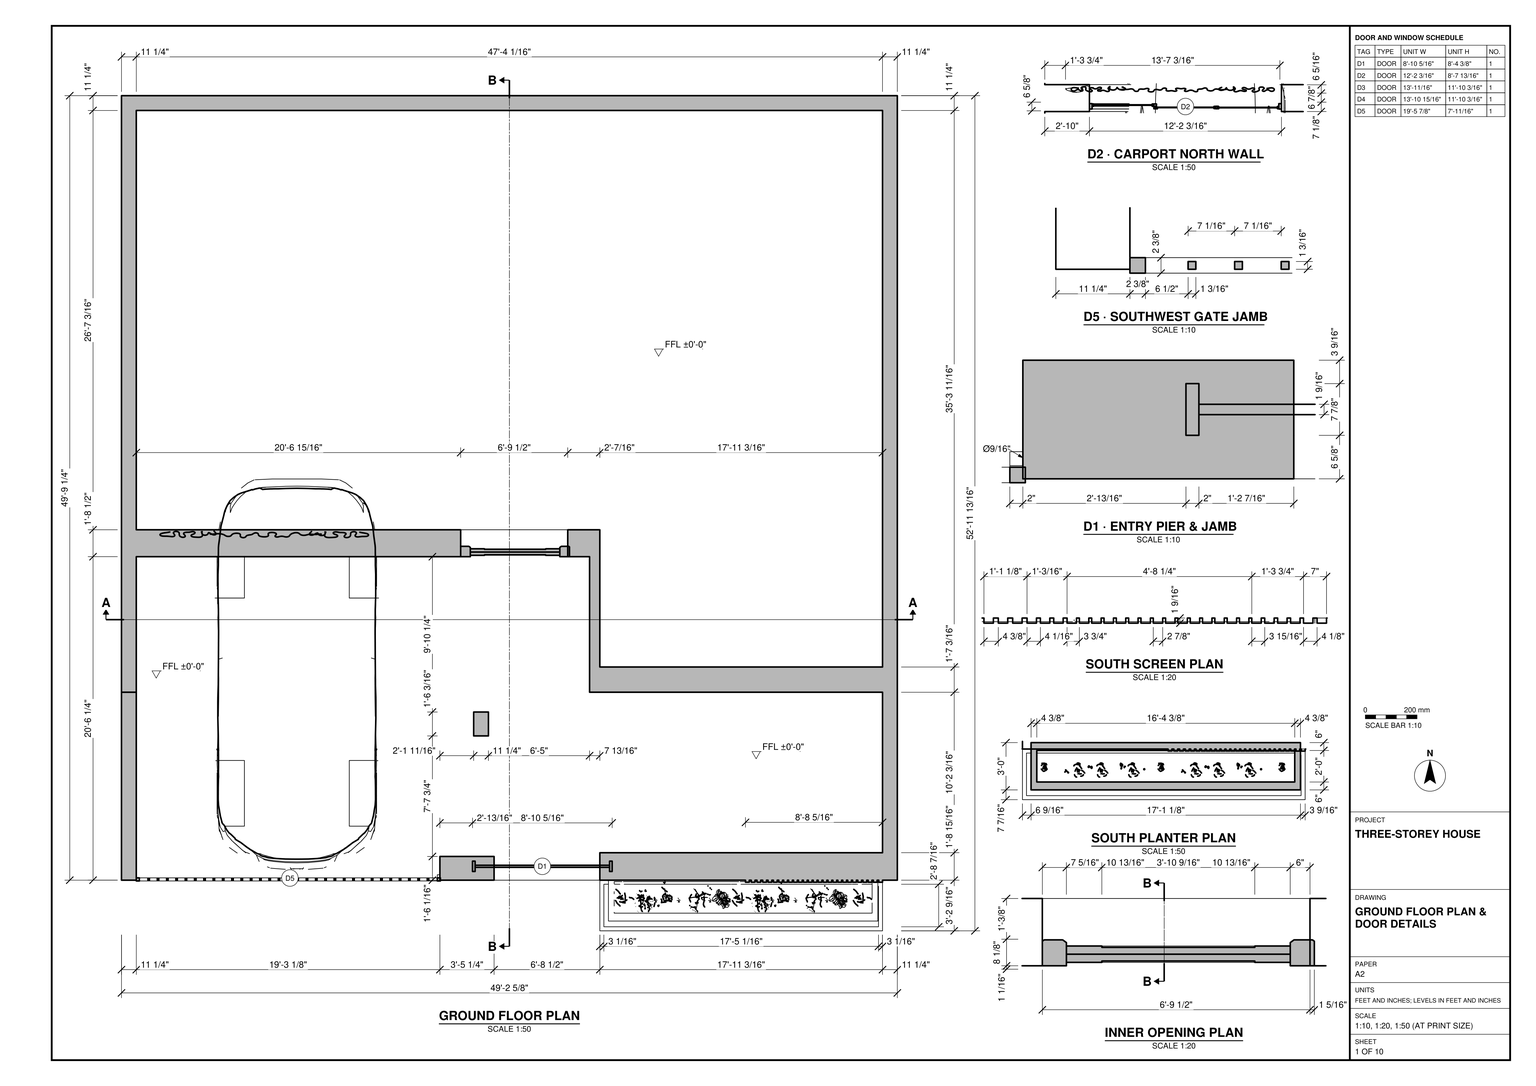
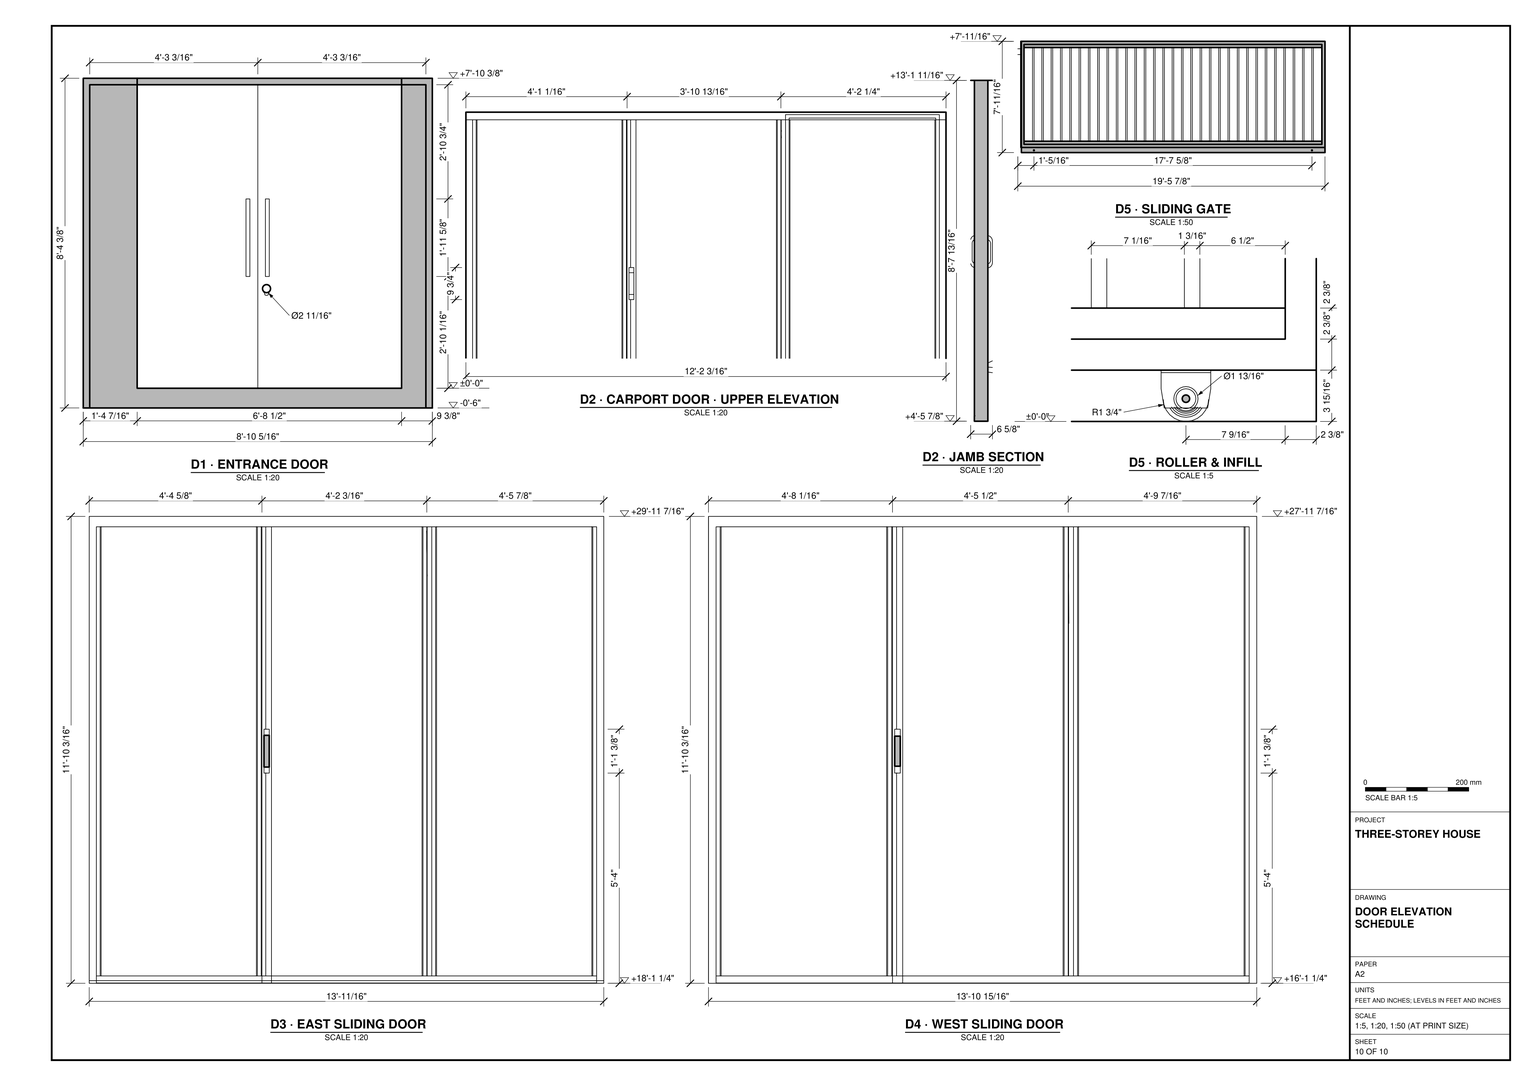
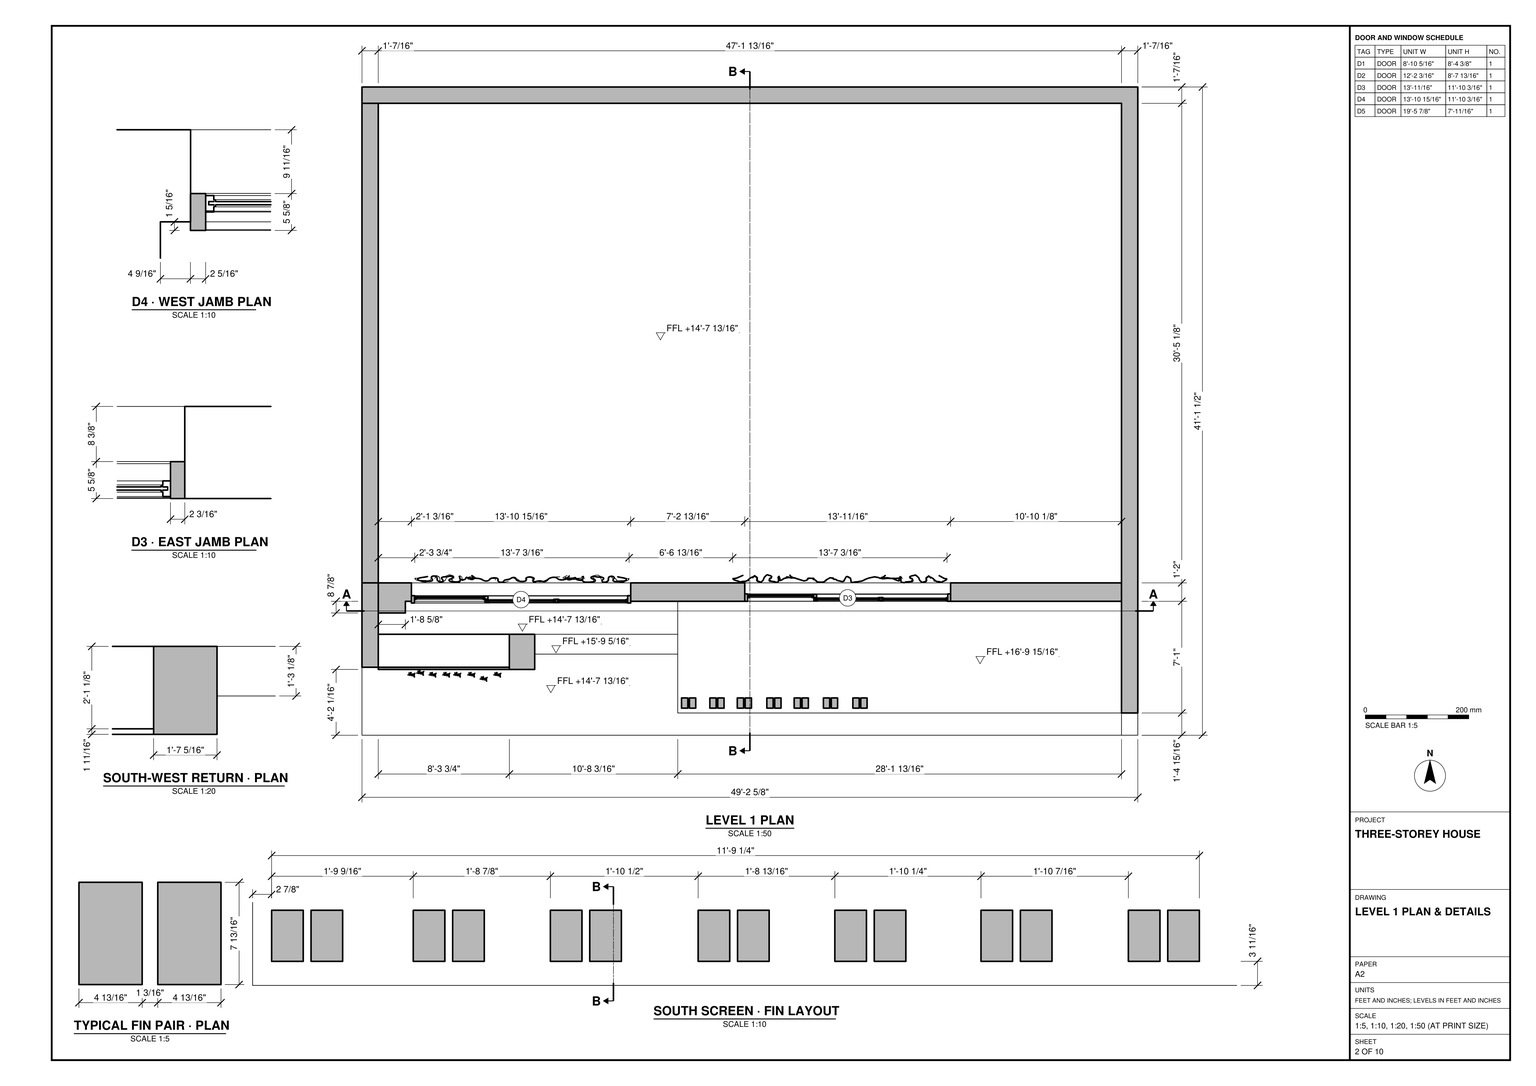
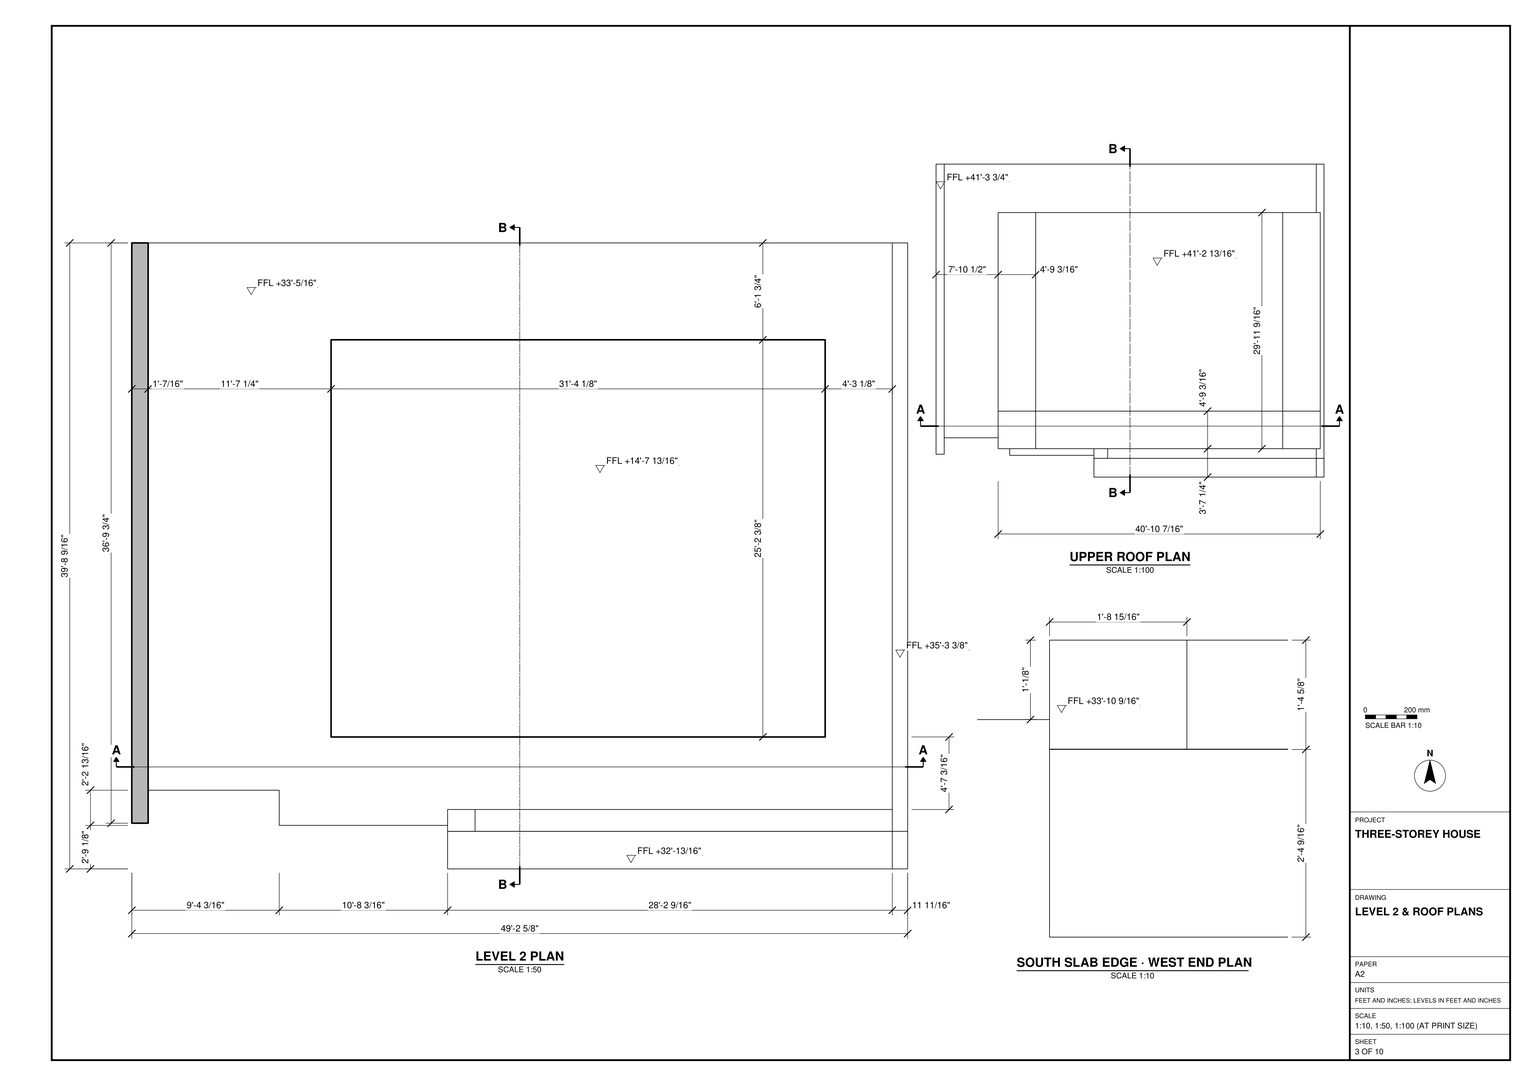
Build the three-storey house in SketchUp from task_files/diagram_01.pdf. Work in feet and inches. Set out the full model to measure 49'-2 5/8" across the frontage, 52'-11 13/16" from front to back and 41'-9 3/4" high. Use the finished floor levels ±0'-0", +14'-7 13/16" and +33'-5/16".

Use the south frontage to align the plans. Place the carport at the southwest, with its sliding gate facing the street, the separate entrance to its east and the projecting planter farther east. Follow the drawn wall thicknesses, returns and opening positions rather than using a uniform wall thickness throughout. Fit the entrance leaves, carport door, sliding doors and gate to their respective openings using the plan details and door elevations.

On the level above the carport, set the wall with the east and west sliding doors back from the terrace edge. Model the changes in terrace level, the southwest return and the paired vertical screen fins. Follow the plans and sections for the floor slabs, roof profile, and any stairs, built-in joinery or main furniture shown. Place a car in the carport and planting in the south planter. Decor and loose items may be any suitable library components.

Keep shell elements and individual furniture or joinery pieces in separate groups or components, and use components for repeated parts. Save one SketchUp model as output_files/three_storey_house_with_a_carport_and_screened_terrace.skp.

# SketchUp Ruby script. Lengths in inches.
U = 1.inch
M = Sketchup.active_model
def pt(a) = Geom::Point3d.new(a.map { |v| v * U })
def face(e, loops, mat)
  f = e.add_face(loops[0].map { |a| pt(a) })
  loops[1..].each { |l| e.add_face(l.map { |a| pt(a) }).erase! }
  f.material = f.back_material = mat if mat
  f
end
# faces: each face lists its corners as indices into pts; further lists are holes
def faces(e, pts, list, mat = nil) = list.each { |f| face(e, (f[0].is_a?(Array) ? f : [f]).map { |l| l.map { |i| pts[i] } }, mat) }
# xy, xz, yz: faces in a plane at the given z, y or x. An outline is a flat list of corners, or four numbers for a rectangle; further outlines are holes
def ring(l) = l.size == 4 ? [[l[0], l[1]], [l[2], l[1]], [l[2], l[3]], [l[0], l[3]]] : l.each_slice(2).to_a
def flat(e, list, mat, &to3) = list.each { |f| face(e, (f[0].is_a?(Array) ? f : [f]).map { |l| ring(l).map { |u, v| to3.(u, v) } }, mat) }
def xy(e, z, list, mat = nil) = flat(e, list, mat) { |x, y| [x, y, z] }
def xz(e, y, list, mat = nil) = flat(e, list, mat) { |x, z| [x, y, z] }
def yz(e, x, list, mat = nil) = flat(e, list, mat) { |y, z| [x, y, z] }
def lines(e, pts, list) = list.each { |a, b| e.add_line(pt(pts[a]), pt(pts[b])) }
# prism: a flat outline (further loops are holes) pulled along v
def prism(e, loops, v, mat = nil)
  f = face(e, loops, mat); d = Geom::Vector3d.new(v.map { |x| x * U })
  f.pushpull(f.normal.samedirection?(d) ? d.length : -d.length)
end
def box(e, o, s, mat = nil) = prism(e, [[o, [o[0] + s[0], o[1], o[2]], [o[0] + s[0], o[1] + s[1], o[2]], [o[0], o[1] + s[1], o[2]]]], [0, 0, s[2]], mat)
def at(x, y, z, deg = 0) = Geom::Transformation.translation(pt([x, y, z])) * Geom::Transformation.rotation(ORIGIN, Z_AXIS, deg.degrees)
def axes(o, x, y, z) = Geom::Transformation.new([*x, 0, *y, 0, *z, 0, *pt(o).to_a, 1])
def part(name) = M.definitions.add(name)
# library, detail: a bought-in or finely detailed component or shape, given as its bounding box
def library(name, o, s) = part(name).tap { |d| box(d.entities, o, s) }
def detail(e, o, s) = box(e.add_group.entities, o, s)
def put(e, d, t, mat = nil) = e.add_instance(d, t).tap { |i| i.material = mat if mat }
def group(e, t, mat = nil) = e.add_group.tap { |g| g.transformation = t; g.material = mat if mat }.entities
root = M.entities
M.materials.add("Material__1").color = [95, 70, 46]
M.materials.add("[0130_Gainsboro]").color = [220, 220, 220]
M.materials.add("[0132_LightGray]").color = [169, 169, 169]
M.materials.add("[Field Rectangle Tile]").color = [196, 189, 179]
M.materials.add("[Granite Dark Gray]").color = [69, 68, 68]
M.materials.add("[Wood Veneer 01]").color = [120, 70, 37]
c1 = library("Group5_1",[-7.56,-66.38,0.11],[6.33,135.04,120.95])
c2 = library("Sliding Door",[0,0,0],[94.49,5.83,91.73])
c3 = library("元件\#5",[-4.39,0,0],[5.37,35.83,90.55])
c4 = library("2016+Honda+Civic+LX+Sedan+(1)",[0.01,0.03,0.02],[16.17,34.46,10.62])
c5 = library("Sliding Gate",[0,0,0],[194.88,4.13,70.58])
c6 = library("door (3)",[-4.72,-1.97,0],[7.87,106.3,100.39])
c7 = library("Potted trailing plant",[-13.52,-13.75,-7.41],[40.56,40.5625,37.31])
c8 = library("Areca palm plant",[0,0,0],[49.1,36.6,54.46])
c9 = library("Group\#74",[-84.69,-90.07,-0.36],[176.51,175.13,171.4])
c10 = library("Group38\#2",[14.01,28.44,-23.43],[18.58,18.32,38.89])
c11 = library("Group20\#1",[-20.81,-17.08,3.79],[39.86,39.43,37.51])
c12 = library("Group\#130",[-7.34,-1.2,0],[38.67,35.81,49.04])
xy(root,-6,[[0,38.5625,590.625,635.8125]])
xy(root,0,[[364.15,0,579.35,38.5625],[[11.28,38.5625,242.39,38.5625,242.39,56.625,283.64,56.625,283.64,38.5625,364.15,38.5625,364.15,59.47,579.35,59.47,579.35,181.65,356.34,181.65,356.34,284.84,339.71,284.84,339.71,305.33,258.21,305.33,258.21,284.84,11.28,284.84],[268.1,148.39,279.35,166.59]],[0,181.65,11.28,181.65,11.28,284.84,258.21,284.84,258.21,305.33,11.28,305.33,11.28,624.53,579.35,624.53,579.35,200.85,364.15,200.85,364.15,305.33,339.71,305.33,339.71,284.84,356.34,284.84,356.34,181.65,590.625,181.65,590.625,635.8125,0,635.8125],[364.15,200.85,579.35,200.85,579.35,624.53,11.28,624.53,11.28,305.33,364.15,305.33],[364.15,200.85,579.35,200.85,579.35,624.53,11.28,624.53,11.28,305.33,364.15,305.33]])
xy(root,7.6875,[[367.23,3.08,576.27,3.08,576.27,33.92,574.36,33.92,574.36,35.49,367.23,35.49]])
xy(root,33.625,[[[364.15,0,579.35,0,579.35,37,576.47,37,576.47,38.5625,575.22,38.5625,575.22,37,572.35,37,572.35,38.5625,571.28,38.5625,571.28,37,568.41,37,568.41,38.5625,567.35,38.5625,567.35,37,564.47,37,564.47,38.5625,563.41,38.5625,563.41,37,560.53,37,560.53,38.5625,559.47,38.5625,559.47,37,556.6,37,556.6,38.5625,555.72,38.5625,555.72,37,552.85,37,552.85,38.5625,551.97,38.5625,551.97,37,549.1,37,549.1,38.5625,548.22,38.5625,548.22,37,545.35,37,545.35,38.5625,544.47,38.5625,544.47,37,541.6,37,541.6,38.5625,540.72,38.5625,540.72,37,537.85,37,537.85,38.5625,536.97,38.5625,536.97,37,534.1,37,534.1,38.5625,533.22,38.5625,533.22,37,530.35,37,530.35,38.5625,529.47,38.5625,529.47,37,526.6,37,526.6,38.5625,525.72,38.5625,525.72,37,522.85,37,522.85,38.5625,521.97,38.5625,521.97,37,519.1,37,519.1,38.5625,518.22,38.5625,518.22,37,515.35,37,515.35,38.5625,514.47,38.5625,514.47,37,511.6,37,511.6,38.5625,510.72,38.5625,510.72,37,507.85,37,507.85,38.5625,506.97,38.5625,506.97,37,504.1,37,504.1,38.5625,503.22,38.5625,503.22,37,500.35,37,500.35,38.5625,499.16,38.5625,499.16,37,496.28,37,496.28,38.5625,495.1,38.5625,495.1,37,492.22,37,492.22,38.5625,491.03,38.5625,491.03,37,488.16,37,488.16,38.5625,486.66,38.5625,486.66,37,483.78,37,483.78,38.5625,482.28,38.5625,482.28,37,479.41,37,479.41,38.5625,477.91,38.5625,477.91,37,475.03,37,475.03,38.5625,364.15,38.5625],[367.23,3.08,367.23,35.49,574.36,35.49,574.36,33.92,576.27,33.92,576.27,3.08]],[475.03,37,477.91,38.5625],[479.41,37,482.28,38.5625],[483.78,37,486.66,38.5625],[488.16,37,491.03,38.5625],
  [492.22,37,495.1,38.5625],[496.28,37,499.16,38.5625],[500.35,37,503.22,38.5625],[504.1,37,506.97,38.5625],[507.85,37,510.72,38.5625],
  [511.6,37,514.47,38.5625],[515.35,37,518.22,38.5625],[519.1,37,521.97,38.5625],[522.85,37,525.72,38.5625],[526.6,37,529.47,38.5625],
  [530.35,37,533.22,38.5625],[534.1,37,536.97,38.5625],[537.85,37,540.72,38.5625],[541.6,37,544.47,38.5625],[545.35,37,548.22,38.5625],
  [549.1,37,551.97,38.5625],[552.85,37,555.72,38.5625],[556.6,37,559.47,38.5625],[560.53,37,563.41,38.5625],[564.47,37,567.35,38.5625],
  [568.41,37,571.28,38.5625],[572.35,37,575.22,38.5625],[576.47,37,579.35,38.5625]])
xy(root,53.59,[[45.25,284.84,191.44,305.33]])
xy(root,106.375,[[475.03,37,477.91,37,477.91,38.5625,479.41,38.5625,479.41,37,482.28,37,482.28,38.5625,483.78,38.5625,483.78,37,486.66,37,486.66,38.5625,488.16,38.5625,488.16,37,491.03,37,491.03,38.5625,492.22,38.5625,492.22,37,495.1,37,495.1,38.5625,496.28,38.5625,496.28,37,499.16,37,499.16,38.5625,500.35,38.5625,500.35,37,503.22,37,503.22,38.5625,504.1,38.5625,504.1,37,506.97,37,506.97,38.5625,507.85,38.5625,507.85,37,510.72,37,510.72,38.5625,511.6,38.5625,511.6,37,514.47,37,514.47,38.5625,515.35,38.5625,515.35,37,518.22,37,518.22,38.5625,519.1,38.5625,519.1,37,521.97,37,521.97,38.5625,522.85,38.5625,522.85,37,525.72,37,525.72,38.5625,526.6,38.5625,526.6,37,529.47,37,529.47,38.5625,530.35,38.5625,530.35,37,533.22,37,533.22,38.5625,534.1,38.5625,534.1,37,536.97,37,536.97,38.5625,537.85,38.5625,537.85,37,540.72,37,540.72,38.5625,541.6,38.5625,541.6,37,544.47,37,544.47,38.5625,545.35,38.5625,545.35,37,548.22,37,548.22,38.5625,549.1,38.5625,549.1,37,551.97,37,551.97,38.5625,552.85,38.5625,552.85,37,555.72,37,555.72,38.5625,556.6,38.5625,556.6,37,559.47,37,559.47,38.5625,560.53,38.5625,560.53,37,563.41,37,563.41,38.5625,564.47,38.5625,564.47,37,567.35,37,567.35,38.5625,568.41,38.5625,568.41,37,571.28,37,571.28,38.5625,572.35,38.5625,572.35,37,575.22,37,575.22,38.5625,576.47,38.5625,576.47,37,579.35,37,579.35,59.47,364.15,59.47,364.15,38.5625,475.03,38.5625],[0,38.5625,11.28,181.65],[242.39,38.5625,283.64,56.625],[579.35,38.5625,590.625,181.65]])
xy(root,155.5625,[[0,148.39,11.28,181.65],[11.28,148.39,11.28,284.84,356.34,284.84,356.34,148.39,279.35,148.39,279.35,166.59,268.1,166.59,268.1,148.39],[356.34,148.39,364.15,181.65],[364.15,148.39,590.625,181.65]])
xy(root,157.25,[[258.21,284.84,339.71,305.33]])
xy(root,157.66,[[45.25,284.84,191.44,305.33]])
xy(root,169.8125,[[[0,181.65,0,635.8125,590.625,635.8125,590.625,181.65,356.34,181.65,356.34,284.84,11.28,284.84,11.28,181.65],[364.15,200.85,579.35,200.85,579.35,624.53,11.28,624.53,11.28,305.33,364.15,305.33]]])
xy(root,171.6875,[[0,142.32,590.625,148.39]])
xy(root,175.8125,[[0,142.32,578.2,142.32,578.2,204.07,131.51,204.07,131.51,192.39,12.42,192.39,12.42,194.07,0,194.07],[578.2,142.32,590.625,219.17],[0,194.07,12.42,258.3],[12.42,219.17,578.2,219.17,578.2,244.27,33.05,244.27,33.05,235.4,12.42,235.4],[578.2,219.17,590.625,244.27],
  [12.42,235.4,33.05,235.4,33.05,244.27,578.2,244.27,578.2,258.3,12.42,258.3],[0,258.3,12.42,303.21],[12.42,258.3,578.2,623.39],[0,303.21,12.42,623.39]])
xy(root,189.28,[[240.375,181.65,285.45,204.07],[285.45,181.65,578.2,204.07],[12.42,194.07,112.2,219.17],[131.51,204.07,240.375,219.17],[240.375,204.07,285.45,219.17],
  [285.45,204.07,578.2,219.17],[240.375,219.17,285.45,244.27],[285.45,219.17,578.2,244.27]])
xy(root,189.28,[[240.375,159.26,285.45,181.65],[285.45,159.26,578.2,181.65]],"[Granite Dark Gray]")
xy(root,189.49,[[578.2,159.26,590.625,181.65],[578.2,181.65,590.625,244.27]])
xy(root,193.23,[[37.65,244.27,204.59,258.3]])
xy(root,201.91,[[[240.375,159.26,578.2,244.27],[243.27,162.92,248.08,170.71],[249.27,162.92,254.08,170.71],[264.83,162.92,269.64,170.71],[270.83,162.92,275.64,170.71],[285.71,162.92,290.52,170.71],[291.71,162.92,296.52,170.71],[308.21,162.92,313.02,170.71],[314.21,162.92,319.02,170.71],[329.02,162.92,333.83,170.71],[335.02,162.92,339.83,170.71],[351.27,162.92,356.08,170.71],[357.27,162.92,362.08,170.71],[373.71,162.92,378.52,170.71],[379.71,162.92,384.52,170.71]]])
xy(root,218.08,[[291.41,244.27,448.1,258.3]])
xy(root,233.16,[[12.42,194.07,112.2,219.17]])
xy(root,235.85,[[12.42,192.39,112.2,194.07]])
xy(root,335.41,[[37.65,244.27,204.59,258.3]])
xy(root,359.46,[[291.41,244.27,448.1,258.3]])
xy(root,369.9375,[[[240.375,159.26,578.2,187.89],[485.96,166.9,487.51,167.125,488.95,167.74,490.18,168.71,491.12,169.97,491.7,171.42,491.88,172.98,491.66,174.53,491.04,175.97,490.07,177.2,488.82,178.13,487.36,178.71,485.81,178.9,484.26,178.67,482.82,178.06,481.59,177.09,480.65,175.83,480.07,174.38,479.88,172.82,480.11,171.27,480.73,169.83,481.69,168.6,482.95,167.67,484.4,167.08],[393.96,166.9,395.51,167.125,396.95,167.74,398.18,168.71,399.12,169.97,399.7,171.42,399.88,172.98,399.66,174.53,399.04,175.97,398.07,177.2,396.82,178.13,395.36,178.71,393.81,178.9,392.26,178.67,390.82,178.06,389.59,177.09,388.65,175.83,388.07,174.38,387.88,172.82,388.11,171.27,388.73,169.83,389.69,168.6,390.95,167.67,392.4,167.08],[243.27,162.92,248.08,170.71],[249.27,162.92,254.08,170.71],[264.83,162.92,269.64,170.71],[270.83,162.92,275.64,170.71],[285.71,162.92,290.52,170.71],[291.71,162.92,296.52,170.71],[308.21,162.92,313.02,170.71],[314.21,162.92,319.02,170.71],[329.02,162.92,333.83,170.71],[335.02,162.92,339.83,170.71],[351.27,162.92,356.08,170.71],[357.27,162.92,362.08,170.71],[373.71,162.92,378.52,170.71],[379.71,162.92,384.52,170.71]]])
xy(root,372.63,[[240.375,159.26,578.2,161.57],[578.2,159.26,579.125,161.57]])
xy(root,372.8125,[[393.96,166.9,392.4,167.08,390.95,167.67,389.69,168.6,388.73,169.83,388.11,171.27,387.88,172.82,388.07,174.38,388.65,175.83,389.59,177.09,390.82,178.06,392.26,178.67,393.81,178.9,395.36,178.71,396.82,178.13,398.07,177.2,399.04,175.97,399.66,174.53,399.88,172.98,399.7,171.42,399.12,169.97,398.18,168.71,396.95,167.74,395.51,167.125],[485.96,166.9,484.4,167.08,482.95,167.67,481.69,168.6,480.73,169.83,480.11,171.27,479.88,172.82,480.07,174.38,480.65,175.83,481.59,177.09,482.82,178.06,484.26,178.67,485.81,178.9,487.36,178.71,488.82,178.13,490.07,177.2,491.04,175.97,491.66,174.53,491.88,172.98,491.7,171.42,491.12,169.97,490.18,168.71,488.95,167.74,487.51,167.125]])
xy(root,378.8125,[[578.2,181.65,590.625,187.89],[578.2,187.89,578.2,623.39,0,623.39,0,635.8125,590.625,635.8125,590.625,187.89],[240.375,187.89,240.375,192.39,131.51,192.39,131.51,219.17,12.42,219.17,12.42,235.4,22.74,235.4,22.74,227.71,238.08,227.71,238.08,235.4,33.05,235.4,33.05,244.27,578.2,244.27,578.2,187.89],[0,219.17,12.42,258.3],[22.74,227.71,25.42,235.4],
  [25.42,227.71,238.08,235.4],[12.42,235.4,12.42,258.3,578.2,258.3,578.2,244.27,33.05,244.27,33.05,235.4],[0,258.3,12.42,303.21],[12.42,258.3,578.2,623.39],[0,303.21,12.42,623.39]])
xy(root,381.44,[[240.375,159.26,578.91,161.57],[578.91,159.26,579.125,161.57]])
xy(root,384.8125,[[240.375,159.26,578.91,187.84],[240.375,187.84,578.91,187.89],[261.29,187.89,578.91,204.48],[0,219.17,12.42,635.8125]])
xy(root,396.3125,[[240.375,187.89,261.29,204.48],[[112.2,192.39,240.375,192.39,240.375,204.48,578.91,204.48,578.91,635.8125,12.42,635.8125,12.42,219.17,112.2,219.17],[151.68,259.69,527.8,562.07]]])
xy(root,406.5625,[[240.375,187.84,261.29,204.48]])
xy(root,423.375,[[578.91,159.26,590.625,187.89],[578.91,187.89,590.625,635.8125]])
xy(root,475.25,[[117.45,225.46,117.45,539.13,128.74,539.13,128.74,236.76,550.74,236.76,550.74,539.13,562.03,539.13,562.03,225.46],[151.68,259.69,527.8,562.07]])
xy(root,475.25,[[[94.52,202.53,94.52,562.07,151.68,562.07,151.68,259.69,527.8,259.69,527.8,562.07,584.97,562.07,584.97,202.53],[117.45,225.46,562.03,225.46,562.03,539.13,550.74,539.13,550.74,236.76,128.74,236.76,128.74,539.13,117.45,539.13]]],"[Wood Veneer 01]")
xy(root,477.58,[[94.52,202.53,101.33,562.07]])
xy(root,479.24,[[101.33,202.53,584.97,209.34]],"[Granite Dark Gray]")
xy(root,479.9,[[583.91,209.34,584.97,562.07]])
xy(root,491.3,[[94.52,209.34,101.33,562.07],[583.91,209.34,584.97,562.07]])
xy(root,491.3,[[94.52,202.53,584.97,209.34]],"[Granite Dark Gray]")
xy(root,494.8125,[[94.52,202.53,151.68,259.69],[527.8,202.53,584.97,259.69],[94.52,259.69,151.68,562.07],[151.68,259.69,527.8,562.07],[527.8,259.69,584.97,562.07]])
xy(root,494.8125,[[151.68,202.53,527.8,259.69]],"[Granite Dark Gray]")
xy(root,495.75,[[0,194.07,12.42,635.8125]])
xz(root,0,[[364.15,0,579.35,33.625]])
xz(root,3.08,[[367.23,7.6875,576.27,33.625]])
xz(root,33.92,[[574.36,7.6875,576.27,33.625]])
xz(root,35.49,[[367.23,7.6875,574.36,33.625]])
xz(root,37,[[475.03,33.625,477.91,106.375],[479.41,33.625,482.28,106.375],[483.78,33.625,486.66,106.375],[488.16,33.625,491.03,106.375],[492.22,33.625,495.1,106.375],
  [496.28,33.625,499.16,106.375],[500.35,33.625,503.22,106.375],[504.1,33.625,506.97,106.375],[507.85,33.625,510.72,106.375],[511.6,33.625,514.47,106.375],
  [515.35,33.625,518.22,106.375],[519.1,33.625,521.97,106.375],[522.85,33.625,525.72,106.375],[526.6,33.625,529.47,106.375],[530.35,33.625,533.22,106.375],
  [534.1,33.625,536.97,106.375],[537.85,33.625,540.72,106.375],[541.6,33.625,544.47,106.375],[545.35,33.625,548.22,106.375],[549.1,33.625,551.97,106.375],
  [552.85,33.625,555.72,106.375],[556.6,33.625,559.47,106.375],[560.53,33.625,563.41,106.375],[564.47,33.625,567.35,106.375],[568.41,33.625,571.28,106.375],
  [572.35,33.625,575.22,106.375],[576.47,33.625,579.35,106.375]],"[Wood Veneer 01]")
xz(root,38.5625,[[0,-6,590.625,-6,590.625,0,283.64,0,283.64,74.62,242.77,74.62,242.77,79.01,283.64,79.01,283.64,106.375,242.39,106.375,242.39,0,11.28,0,11.28,106.375,0,106.375],[364.15,0,579.35,33.625],[579.35,0,590.625,106.375],[364.15,33.625,475.03,106.375]])
xz(root,38.5625,[[242.77,74.62,283.64,79.01]],"[Granite Dark Gray]")
xz(root,38.5625,[[477.91,33.625,479.41,106.375],[482.28,33.625,483.78,106.375],[486.66,33.625,488.16,106.375],[491.03,33.625,492.22,106.375],[495.1,33.625,496.28,106.375],
  [499.16,33.625,500.35,106.375],[503.22,33.625,504.1,106.375],[506.97,33.625,507.85,106.375],[510.72,33.625,511.6,106.375],[514.47,33.625,515.35,106.375],
  [518.22,33.625,519.1,106.375],[521.97,33.625,522.85,106.375],[525.72,33.625,526.6,106.375],[529.47,33.625,530.35,106.375],[533.22,33.625,534.1,106.375],
  [536.97,33.625,537.85,106.375],[540.72,33.625,541.6,106.375],[544.47,33.625,545.35,106.375],[548.22,33.625,549.1,106.375],[551.97,33.625,552.85,106.375],
  [555.72,33.625,556.6,106.375],[559.47,33.625,560.53,106.375],[563.41,33.625,564.47,106.375],[567.35,33.625,568.41,106.375],[571.28,33.625,572.35,106.375],
  [575.22,33.625,576.47,106.375]],"[Wood Veneer 01]")
xz(root,56.625,[[242.39,0,283.64,106.375]])
xz(root,59.47,[[364.15,0,579.35,106.375]])
xz(root,142.32,[[0,171.6875,590.625,175.8125]],"[Granite Dark Gray]")
xz(root,148.39,[[268.1,0,279.35,0,279.35,155.5625,590.625,155.5625,590.625,171.6875,0,171.6875,0,155.5625,268.1,155.5625]],"[Granite Dark Gray]")
xz(root,159.26,[[578.2,189.49,590.625,189.49,590.625,423.375,578.91,423.375,578.91,381.44,579.125,381.44,579.125,372.63,578.2,372.63]])
xz(root,159.26,[[240.375,189.28,578.2,201.91],[240.375,369.9375,578.2,372.63],[240.375,381.44,578.91,384.8125]],"[Granite Dark Gray]")
xz(root,161.57,[[240.375,372.63,579.125,381.44]],"[Granite Dark Gray]")
xz(root,162.92,[[243.27,201.91,248.08,369.9375],[249.27,201.91,254.08,369.9375],[264.83,201.91,269.64,369.9375],[270.83,201.91,275.64,369.9375],[285.71,201.91,290.52,369.9375],
  [291.71,201.91,296.52,369.9375],[308.21,201.91,313.02,369.9375],[314.21,201.91,319.02,369.9375],[329.02,201.91,333.83,369.9375],[335.02,201.91,339.83,369.9375],
  [351.27,201.91,356.08,369.9375],[357.27,201.91,362.08,369.9375],[373.71,201.91,378.52,369.9375],[379.71,201.91,384.52,369.9375]],"[Wood Veneer 01]")
xz(root,166.59,[[268.1,0,279.35,155.5625]])
xz(root,170.71,[[243.27,201.91,248.08,369.9375],[249.27,201.91,254.08,369.9375],[264.83,201.91,269.64,369.9375],[270.83,201.91,275.64,369.9375],[285.71,201.91,290.52,369.9375],
  [291.71,201.91,296.52,369.9375],[308.21,201.91,313.02,369.9375],[314.21,201.91,319.02,369.9375],[329.02,201.91,333.83,369.9375],[335.02,201.91,339.83,369.9375],
  [351.27,201.91,356.08,369.9375],[357.27,201.91,362.08,369.9375],[373.71,201.91,378.52,369.9375],[379.71,201.91,384.52,369.9375]])
xz(root,181.65,[[0,0,11.28,106.375],[356.34,0,364.15,155.5625],[0,106.375,11.28,155.5625],[0,155.5625,11.28,169.8125],[356.34,155.5625,364.15,169.8125],
  [364.15,155.5625,590.625,169.8125]])
xz(root,181.65,[[364.15,0,579.35,0,579.35,106.375,590.625,106.375,590.625,155.5625,364.15,155.5625]],"[Field Rectangle Tile]")
xz(root,187.84,[[240.375,384.8125,578.91,384.8125,578.91,416.875,261.29,406.5625,240.375,406.5625]],"[0132_LightGray]")
xz(root,187.89,[[240.375,369.9375,578.2,378.8125],[240.375,384.8125,261.29,396.3125]])
xz(root,192.39,[[112.2,175.8125,131.51,175.8125,131.51,378.8125,240.375,378.8125,240.375,396.3125,112.2,396.3125]],"[0132_LightGray]")
xz(root,192.39,[[12.42,175.8125,112.2,235.85]],"[Granite Dark Gray]")
xz(root,194.07,[[12.42,175.8125,112.2,189.28],[12.42,189.28,112.2,233.16],[12.42,233.16,112.2,235.85]])
xz(root,194.07,[[0,175.8125,12.42,495.75]],"[0132_LightGray]")
xz(root,200.85,[[364.15,0,579.35,169.8125]])
xz(root,202.53,[[94.52,475.25,584.97,475.25,584.97,479.24,101.33,479.24,101.33,477.58,94.52,477.58],[94.52,491.3,584.97,494.8125]],"[Granite Dark Gray]")
xz(root,204.07,[[131.51,175.8125,578.2,189.28]],"[0130_Gainsboro]")
xz(root,204.48,[[261.29,384.8125,578.91,396.3125],[240.375,396.3125,240.375,406.5625,261.29,406.5625,578.91,416.875,578.91,396.3125]])
xz(root,209.34,[[101.33,479.24,584.97,479.24,584.97,479.9,583.91,479.9,583.91,491.3,101.33,491.3]],"[Granite Dark Gray]")
xz(root,219.17,[[12.42,175.8125,12.42,189.28,112.2,189.28,112.2,378.8125,131.51,378.8125,131.51,189.28,578.2,189.28,578.2,175.8125],[12.42,189.28,112.2,233.16],[0,378.8125,12.42,384.8125]])
xz(root,219.17,[[12.42,378.8125,112.2,396.3125]],"[0132_LightGray]")
xz(root,235.4,[[12.42,175.8125,33.05,378.8125]],"[Granite Dark Gray]")
xz(root,244.27,[[578.2,175.8125,590.625,189.49],[240.375,189.28,285.45,201.91]])
xz(root,244.27,[[[33.05,175.8125,578.2,175.8125,578.2,189.28,240.375,189.28,240.375,201.91,578.2,201.91,578.2,378.8125,33.05,378.8125],[37.65,193.23,204.59,335.41],[291.41,218.08,448.1,359.46]]],"[Field Rectangle Tile]")
xz(root,258.3,[[0,175.8125,12.42,378.8125],[[12.42,175.8125,578.2,378.8125],[37.65,193.23,204.59,335.41],[291.41,218.08,448.1,359.46]]])
xz(root,259.69,[[151.68,475.25,527.8,494.8125]])
xz(root,259.69,[[151.68,396.3125,527.8,475.25]],"[0132_LightGray]")
xz(root,284.84,[[339.71,0,356.34,155.5625],[11.28,155.5625,45.25,155.5625,45.25,157.66,191.44,157.66,191.44,155.5625,258.21,155.5625,258.21,157.25,339.71,157.25,339.71,155.5625,356.34,155.5625,356.34,169.8125,11.28,169.8125],[45.25,155.5625,191.44,157.66],[258.21,155.5625,339.71,157.25]])
xz(root,284.84,[[11.28,0,258.21,0,258.21,155.5625,191.44,155.5625,191.44,53.59,45.25,53.59,45.25,155.5625,11.28,155.5625]],"[0130_Gainsboro]")
xz(root,305.33,[[[11.28,0,11.28,169.8125,364.15,169.8125,364.15,0,339.71,0,339.71,157.25,258.21,157.25,258.21,0],[45.25,53.59,191.44,157.66]]])
xz(root,562.07,[[151.68,396.3125,527.8,475.25],[94.52,475.25,94.52,477.58,101.33,477.58,101.33,491.3,94.52,491.3,94.52,494.8125,151.68,494.8125,151.68,475.25],[151.68,475.25,527.8,494.8125],[527.8,475.25,527.8,494.8125,584.97,494.8125,584.97,491.3,583.91,491.3,583.91,479.9,584.97,479.9,584.97,475.25]])
xz(root,623.39,[[0,175.8125,12.42,378.8125],[12.42,175.8125,578.2,378.8125]])
xz(root,624.53,[[11.28,0,579.35,169.8125]])
xz(root,635.8125,[[0,-6,590.625,0],[0,0,590.625,169.8125],[0,169.8125,590.625,378.8125],[0,378.8125,0,384.8125,12.42,384.8125,12.42,396.3125,578.91,396.3125,578.91,423.375,590.625,423.375,590.625,378.8125],[0,384.8125,12.42,495.75]])
yz(root,0,[[38.5625,-6,38.5625,106.375,181.65,106.375,181.65,0,635.8125,0,635.8125,-6],[181.65,0,635.8125,169.8125],[148.39,155.5625,148.39,171.6875,142.32,171.6875,142.32,175.8125,623.39,175.8125,623.39,378.8125,635.8125,378.8125,635.8125,169.8125,181.65,169.8125,181.65,155.5625],[194.07,175.8125,194.07,495.75,635.8125,495.75,635.8125,384.8125,219.17,384.8125,219.17,378.8125,258.3,378.8125,258.3,175.8125],[258.3,175.8125,303.21,378.8125],
  [303.21,175.8125,623.39,378.8125],[219.17,378.8125,635.8125,384.8125]])
yz(root,11.28,[[38.5625,0,181.65,106.375],[181.65,0,284.84,155.5625],[305.33,0,624.53,169.8125],[181.65,155.5625,284.84,169.8125]])
yz(root,12.42,[[192.39,175.8125,194.07,235.85],[194.07,175.8125,219.17,189.28],[235.4,175.8125,258.3,378.8125],[258.3,175.8125,623.39,378.8125],[194.07,189.28,219.17,233.16],
  [219.17,384.8125,635.8125,396.3125]])
yz(root,12.42,[[219.17,175.8125,235.4,175.8125,235.4,378.8125,219.17,378.8125,219.17,396.3125,635.8125,396.3125,635.8125,495.75,194.07,495.75,194.07,233.16,219.17,233.16]],"[0130_Gainsboro]")
yz(root,33.05,[[235.4,175.8125,244.27,378.8125]],"[Granite Dark Gray]")
yz(root,37.65,[[244.27,193.23,258.3,335.41]])
yz(root,45.25,[[284.84,53.59,305.33,157.66]])
yz(root,94.52,[[202.53,475.25,562.07,477.58],[202.53,491.3,562.07,494.8125]])
yz(root,101.33,[[202.53,477.58,202.53,479.24,209.34,479.24,209.34,491.3,562.07,491.3,562.07,477.58]])
yz(root,112.2,[[192.39,175.8125,194.07,235.85],[194.07,189.28,219.17,233.16],[194.07,233.16,194.07,235.85,192.39,235.85,192.39,378.8125,219.17,378.8125,219.17,233.16],[192.39,378.8125,219.17,396.3125]])
yz(root,131.51,[[192.39,175.8125,204.07,189.28],[192.39,189.28,219.17,378.8125]])
yz(root,151.68,[[259.69,396.3125,562.07,475.25],[259.69,475.25,562.07,494.8125]])
yz(root,191.44,[[284.84,53.59,305.33,157.66]])
yz(root,204.59,[[244.27,193.23,258.3,335.41]])
yz(root,240.375,[[159.26,189.28,181.65,201.91],[181.65,189.28,244.27,201.91],[159.26,369.9375,159.26,372.63,161.57,372.63,161.57,381.44,159.26,381.44,159.26,384.8125,187.89,384.8125,187.89,396.3125,192.39,396.3125,192.39,378.8125,187.89,378.8125,187.89,369.9375],[187.84,384.8125,187.84,406.5625,204.48,406.5625,204.48,396.3125,187.89,396.3125,187.89,384.8125]])
yz(root,242.39,[[38.5625,0,56.625,106.375]])
yz(root,243.27,[[162.92,201.91,170.71,369.9375]])
yz(root,248.08,[[162.92,201.91,170.71,369.9375]])
yz(root,249.27,[[162.92,201.91,170.71,369.9375]])
yz(root,254.08,[[162.92,201.91,170.71,369.9375]])
yz(root,258.21,[[284.84,0,305.33,157.25]])
yz(root,261.29,[[187.89,384.8125,204.48,396.3125]])
yz(root,264.83,[[162.92,201.91,170.71,369.9375]])
yz(root,268.1,[[148.39,0,166.59,155.5625]])
yz(root,269.64,[[162.92,201.91,170.71,369.9375]])
yz(root,270.83,[[162.92,201.91,170.71,369.9375]])
yz(root,275.64,[[162.92,201.91,170.71,369.9375]])
yz(root,279.35,[[148.39,0,166.59,155.5625]])
yz(root,283.64,[[38.5625,0,56.625,106.375]])
yz(root,285.71,[[162.92,201.91,170.71,369.9375]])
yz(root,290.52,[[162.92,201.91,170.71,369.9375]])
yz(root,291.41,[[244.27,218.08,258.3,359.46]])
yz(root,291.71,[[162.92,201.91,170.71,369.9375]])
yz(root,296.52,[[162.92,201.91,170.71,369.9375]])
yz(root,308.21,[[162.92,201.91,170.71,369.9375]])
yz(root,313.02,[[162.92,201.91,170.71,369.9375]])
yz(root,314.21,[[162.92,201.91,170.71,369.9375]])
yz(root,319.02,[[162.92,201.91,170.71,369.9375]])
yz(root,329.02,[[162.92,201.91,170.71,369.9375]])
yz(root,333.83,[[162.92,201.91,170.71,369.9375]])
yz(root,335.02,[[162.92,201.91,170.71,369.9375]])
yz(root,339.71,[[284.84,0,305.33,157.25]])
yz(root,339.83,[[162.92,201.91,170.71,369.9375]])
yz(root,351.27,[[162.92,201.91,170.71,369.9375]])
yz(root,356.08,[[162.92,201.91,170.71,369.9375]])
yz(root,356.34,[[181.65,0,284.84,155.5625],[181.65,155.5625,284.84,169.8125]])
yz(root,357.27,[[162.92,201.91,170.71,369.9375]])
yz(root,362.08,[[162.92,201.91,170.71,369.9375]])
yz(root,364.15,[[0,0,38.5625,33.625],[38.5625,0,59.47,106.375],[200.85,0,305.33,169.8125]])
yz(root,367.23,[[3.08,7.6875,35.49,33.625]])
yz(root,373.71,[[162.92,201.91,170.71,369.9375]])
yz(root,378.52,[[162.92,201.91,170.71,369.9375]])
yz(root,379.71,[[162.92,201.91,170.71,369.9375]])
yz(root,384.52,[[162.92,201.91,170.71,369.9375]])
yz(root,448.1,[[244.27,218.08,258.3,359.46]])
yz(root,475.03,[[37,33.625,37,106.375,38.5625,106.375,38.5625,38.2,37.4375,38.2,37.4375,33.625],[37.4375,33.625,38.5625,38.2]])
yz(root,477.91,[[37,33.625,38.5625,106.375]])
yz(root,479.41,[[37,33.625,38.5625,106.375]])
yz(root,482.28,[[37,33.625,38.5625,106.375]])
yz(root,483.78,[[37,33.625,38.5625,106.375]])
yz(root,486.66,[[37,33.625,38.5625,106.375]])
yz(root,488.16,[[37,33.625,38.5625,106.375]])
yz(root,491.03,[[37,33.625,38.5625,106.375]])
yz(root,492.22,[[37,33.625,38.5625,106.375]])
yz(root,495.1,[[37,33.625,38.5625,106.375]])
yz(root,496.28,[[37,33.625,38.5625,106.375]])
yz(root,499.16,[[37,33.625,38.5625,106.375]])
yz(root,500.35,[[37,33.625,38.5625,106.375]])
yz(root,503.22,[[37,33.625,38.5625,106.375]])
yz(root,504.1,[[37,33.625,38.5625,106.375]])
yz(root,506.97,[[37,33.625,38.5625,106.375]])
yz(root,507.85,[[37,33.625,38.5625,106.375]])
yz(root,510.72,[[37,33.625,38.5625,106.375]])
yz(root,511.6,[[37,33.625,38.5625,106.375]])
yz(root,514.47,[[37,33.625,38.5625,106.375]])
yz(root,515.35,[[37,33.625,38.5625,106.375]])
yz(root,518.22,[[37,33.625,38.5625,106.375]])
yz(root,519.1,[[37,33.625,38.5625,106.375]])
yz(root,521.97,[[37,33.625,38.5625,106.375]])
yz(root,522.85,[[37,33.625,38.5625,106.375]])
yz(root,525.72,[[37,33.625,38.5625,106.375]])
yz(root,526.6,[[37,33.625,38.5625,106.375]])
yz(root,527.8,[[259.69,396.3125,562.07,475.25],[259.69,475.25,562.07,494.8125]])
yz(root,529.47,[[37,33.625,38.5625,106.375]])
yz(root,530.35,[[37,33.625,38.5625,106.375]])
yz(root,533.22,[[37,33.625,38.5625,106.375]])
yz(root,534.1,[[37,33.625,38.5625,106.375]])
yz(root,536.97,[[37,33.625,38.5625,106.375]])
yz(root,537.85,[[37,33.625,38.5625,106.375]])
yz(root,540.72,[[37,33.625,38.5625,106.375]])
yz(root,541.6,[[37,33.625,38.5625,106.375]])
yz(root,544.47,[[37,33.625,38.5625,106.375]])
yz(root,545.35,[[37,33.625,38.5625,106.375]])
yz(root,548.22,[[37,33.625,38.5625,106.375]])
yz(root,549.1,[[37,33.625,38.5625,106.375]])
yz(root,551.97,[[37,33.625,38.5625,106.375]])
yz(root,552.85,[[37,33.625,38.5625,106.375]])
yz(root,555.72,[[37,33.625,38.5625,106.375]])
yz(root,556.6,[[37,33.625,38.5625,106.375]])
yz(root,559.47,[[37,33.625,38.5625,106.375]])
yz(root,560.53,[[37,33.625,38.5625,106.375]])
yz(root,563.41,[[37,33.625,38.5625,106.375]])
yz(root,564.47,[[37,33.625,38.5625,106.375]])
yz(root,567.35,[[37,33.625,38.5625,106.375]])
yz(root,568.41,[[37,33.625,38.5625,106.375]])
yz(root,571.28,[[37,33.625,38.5625,106.375]])
yz(root,572.35,[[37,33.625,38.5625,106.375]])
yz(root,574.36,[[33.92,7.6875,35.49,33.625]])
yz(root,575.22,[[37,33.625,38.5625,106.375]])
yz(root,576.27,[[3.08,7.6875,33.92,33.625]])
yz(root,576.47,[[37,33.625,38.5625,106.375]])
yz(root,578.2,[[204.07,175.8125,219.17,189.28],[244.27,175.8125,258.3,378.8125],[258.3,175.8125,321.42,378.8125],[321.42,175.8125,623.39,378.8125],[159.26,189.28,181.65,189.49],
  [181.65,189.28,244.27,189.49],[159.26,189.49,181.65,201.91],[181.65,189.49,244.27,201.91],[181.65,369.9375,187.89,378.8125]])
yz(root,578.2,[[159.26,201.91,159.26,369.9375,187.89,369.9375,187.89,378.8125,244.27,378.8125,244.27,201.91]],"[0132_LightGray]")
yz(root,578.91,[[159.26,384.8125,159.26,423.375,635.8125,423.375,635.8125,396.3125,204.48,396.3125,204.48,416.875,187.84,416.875,187.84,384.8125],[187.84,384.8125,187.89,416.875],[187.89,384.8125,204.48,416.875]])
yz(root,579.125,[[159.26,372.63,161.57,381.44]])
yz(root,579.35,[[0,0,38.5625,33.625],[59.47,0,181.65,106.375],[200.85,0,624.53,169.8125],[37,33.625,38.5625,106.375]])
yz(root,583.91,[[209.34,479.9,562.07,491.3]])
yz(root,584.97,[[202.53,475.25,562.07,475.25,562.07,479.9,209.34,479.9,209.34,479.24,202.53,479.24],[202.53,491.3,562.07,494.8125]])
yz(root,590.625,[[38.5625,-6,635.8125,-6,635.8125,0,181.65,0,181.65,106.375,38.5625,106.375],[181.65,0,635.8125,169.8125],[148.39,155.5625,181.65,155.5625,181.65,169.8125,635.8125,169.8125,635.8125,378.8125,181.65,378.8125,181.65,189.49,244.27,189.49,244.27,175.8125,142.32,175.8125,142.32,171.6875,148.39,171.6875],[159.26,189.49,181.65,378.8125],[159.26,378.8125,187.89,423.375],
  [187.89,378.8125,635.8125,423.375]])
p = [[475.03,37,81.04],[364.15,38.5625,81.04],[364.15,38.5625,77],[475.03,37,77],[393.96,166.9,369.9375],[392.4,167.08,369.9375],
  [392.4,167.08,372.8125],[393.96,166.9,372.8125],[395.51,167.125,369.9375],[395.51,167.125,372.8125],[485.96,166.9,369.9375],[484.4,167.08,369.9375],
  [484.4,167.08,372.8125],[485.96,166.9,372.8125],[487.51,167.125,369.9375],[487.51,167.125,372.8125],[390.95,167.67,369.9375],[390.95,167.67,372.8125],
  [396.95,167.74,369.9375],[396.95,167.74,372.8125],[482.95,167.67,369.9375],[482.95,167.67,372.8125],[488.95,167.74,369.9375],[488.95,167.74,372.8125],
  [389.69,168.6,369.9375],[389.69,168.6,372.8125],[398.18,168.71,369.9375],[398.18,168.71,372.8125],[481.69,168.6,369.9375],[481.69,168.6,372.8125],
  [490.18,168.71,369.9375],[490.18,168.71,372.8125],[388.73,169.83,369.9375],[388.73,169.83,372.8125],[480.73,169.83,369.9375],[480.73,169.83,372.8125],
  [399.12,169.97,369.9375],[399.12,169.97,372.8125],[491.12,169.97,369.9375],[491.12,169.97,372.8125],[388.11,171.27,369.9375],[388.11,171.27,372.8125],
  [480.11,171.27,369.9375],[480.11,171.27,372.8125],[399.7,171.42,369.9375],[399.7,171.42,372.8125],[491.7,171.42,369.9375],[491.7,171.42,372.8125],
  [387.88,172.82,369.9375],[387.88,172.82,372.8125],[479.88,172.82,369.9375],[479.88,172.82,372.8125],[399.88,172.98,369.9375],[399.88,172.98,372.8125],
  [491.88,172.98,369.9375],[491.88,172.98,372.8125],[388.07,174.38,369.9375],[388.07,174.38,372.8125],[480.07,174.38,369.9375],[480.07,174.38,372.8125],
  [399.66,174.53,369.9375],[399.66,174.53,372.8125],[491.66,174.53,369.9375],[491.66,174.53,372.8125],[388.65,175.83,369.9375],[388.65,175.83,372.8125],
  [480.65,175.83,369.9375],[480.65,175.83,372.8125],[399.04,175.97,369.9375],[399.04,175.97,372.8125],[491.04,175.97,369.9375],[491.04,175.97,372.8125],
  [389.59,177.09,369.9375],[389.59,177.09,372.8125],[481.59,177.09,369.9375],[481.59,177.09,372.8125],[398.07,177.2,369.9375],[398.07,177.2,372.8125],
  [490.07,177.2,369.9375],[490.07,177.2,372.8125],[390.82,178.06,369.9375],[390.82,178.06,372.8125],[482.82,178.06,369.9375],[482.82,178.06,372.8125],
  [396.82,178.13,369.9375],[396.82,178.13,372.8125],[488.82,178.13,369.9375],[488.82,178.13,372.8125],[392.26,178.67,369.9375],[392.26,178.67,372.8125],
  [395.36,178.71,369.9375],[395.36,178.71,372.8125],[484.26,178.67,369.9375],[484.26,178.67,372.8125],[487.36,178.71,369.9375],[487.36,178.71,372.8125],
  [393.81,178.9,369.9375],[393.81,178.9,372.8125],[485.81,178.9,369.9375],[485.81,178.9,372.8125],[261.29,187.84,406.5625],[578.91,187.84,416.875],
  [578.91,187.89,416.875],[578.91,204.48,416.875],[261.29,204.48,406.5625],[242.77,37.97,80.71],[242.77,37.97,77.45]]
faces(root,p,[[0,1,2,3]],"[Granite Dark Gray]")
faces(root,p,[[4,5,6,7],[8,4,7,9],[10,11,12,13],[14,10,13,15],[5,16,17,6],[18,8,9,19],[11,20,21,12],[22,14,15,23],
  [16,24,25,17],[26,18,19,27],[20,28,29,21],[30,22,23,31],[24,32,33,25],[28,34,35,29],[36,26,27,37],[38,30,31,39],
  [32,40,41,33],[34,42,43,35],[44,36,37,45],[46,38,39,47],[40,48,49,41],[42,50,51,43],[52,44,45,53],[54,46,47,55],
  [48,56,57,49],[50,58,59,51],[60,52,53,61],[62,54,55,63],[56,64,65,57],[58,66,67,59],[68,60,61,69],[70,62,63,71],
  [64,72,73,65],[66,74,75,67],[76,68,69,77],[78,70,71,79],[72,80,81,73],[74,82,83,75],[84,76,77,85],[86,78,79,87],
  [80,88,89,81],[90,84,85,91],[82,92,93,83],[94,86,87,95],[88,96,97,89],[96,90,91,97],[92,98,99,93],[98,94,95,99],
  [100,101,102,103,104]])
lines(root,p,[[105,106]])
put(root,c1,axes([362.39,257.07,221.45],[0,-1,0],[1.2084,0,0],[0,0,1.14]))
put(root,c1,axes([120.4,257.07,197.32],[0,-1,0],[1.2084,0,0],[0,0,1.14]))
put(root,c1,axes([107.26,297.63,19.56],[0,-1,0],[1.2084,0,0],[0,0,1.14]))
put(root,c2,axes([37.625,241.07,193.23],[1.767,0,0],[0,1.55,0],[0,0,1.55]))
put(root,c2,axes([291.41,242.38,217.27],[1.65828,0,0],[0,1.55,0],[0,0,1.55]))
put(root,c2,axes([45.25,285.38,53.86],[1.54715,0,0],[0,1.1315,0],[0,0,1.1315]))
put(root,c3,axes([258.21,285.47,3.3125],[0,-1.7,0],[2.312,0,0],[0,0,1.7]))
put(root,c4,axes([63.57,46.03,-0.17],[8.64,0,0],[0,8.64,0],[0,0,8.64]))
put(root,c5,axes([11.28,37.74,0],[1.2,0,0],[0,1.2,0],[0,0,1.2]))
put(root,c6,at(269.2,48.34,-6,-90))
put(root,c7,at(32.9,187.08,224.48))
put(root,c7,at(39.64,188.45,224.48))
put(root,c7,at(49.01,187.08,224.48))
put(root,c7,at(59.45,187.08,224.48))
put(root,c7,at(67.76,187.08,224.48))
put(root,c7,at(78.5,187.08,224.48))
put(root,c7,at(87.85,183.9,224.48))
put(root,c7,at(98.31,187.08,224.48))
g1 = group(root,at(575.8,7.45,23.2))
put(g1,c8,axes([-138.37,-6.2,6.08],[0.49083,0.45017,0],[-0.46283,0.66137,0],[0,0,0.72]))
put(g1,c8,axes([-49.4375,-6.2,6.08],[0.49083,0.45017,0],[-0.46283,0.66137,0],[0,0,0.72]))
put(g1,c9,axes([-168.74,14.93,6.05],[0.07506,-0.04961,0],[0.04333,0.08593,0],[0,0,0.10522]))
put(g1,c9,axes([-127.41,14.93,6.05],[0.07506,-0.04961,0],[0.04333,0.08593,0],[0,0,0.10522]))
put(g1,c9,axes([-62.28,14.93,6.05],[0.07506,-0.04961,0],[0.04333,0.08593,0],[0,0,0.10522]))
put(g1,c9,axes([-151.22,14.93,6.05],[0.07506,-0.04961,0],[0.04333,0.08593,0],[0,0,0.10522]))
put(g1,c10,axes([1.01,-4.1,28.17],[0,0.8848,0],[-0.82698,0,0],[0,0,0.85826]))
put(g1,c9,axes([-38.48,14.93,6.05],[0.07506,-0.04961,0],[0.04333,0.08593,0],[0,0,0.10522]))
put(g1,c9,axes([-105.9,17.19,6.07],[0.12305,-0.08133,0],[0.07104,0.14087,0],[0,0,0.1725]))
put(g1,c9,axes([-79.81,14.93,6.05],[0.07506,-0.04961,0],[0.04333,0.08593,0],[0,0,0.10522]))
put(g1,c11,axes([-69.86,18.97,4.77],[-0.74248,0,0],[0,-0.85,0],[0,0,0.85]))
put(g1,c12,axes([-78.54,24.9375,8],[-0.69007,0,0],[0,-0.79,0],[0,0,0.79]))
put(g1,c9,axes([-13.8,17.19,6.07],[0.12305,-0.08133,0],[0.07104,0.14087,0],[0,0,0.1725]))
g2 = group(g1,at(0,0,0))
xy(g2,0,[[-205.1,0,0,6],[-205.1,30,0,36]])
xy(g2,3,[[-205.1,6,0,30]])
xy(g2,7,[[-200.73,6,-4.37,30]],"Material__1")
xy(g2,15,[[[-205.1,0,0,36],[-200.73,6,-4.37,30]]])
xz(g2,0,[[-205.1,0,0,15]])
xz(g2,6,[[-205.1,0,0,3],[-200.73,7,-4.37,15]])
xz(g2,30,[[-205.1,0,0,3],[-200.73,7,-4.37,15]])
xz(g2,36,[[-205.1,0,0,15]])
yz(g2,-205.1,[[0,0,0,15,36,15,36,0,30,0,30,3,6,3,6,0]])
yz(g2,-200.73,[[6,7,30,15]])
yz(g2,-4.37,[[6,7,30,15]])
yz(g2,0,[[0,0,6,0,6,3,30,3,30,0,36,0,36,15,0,15]])
put(g1,c11,axes([-158.79,18.97,4.77],[-0.74248,0,0],[0,-0.85,0],[0,0,0.85]))
put(g1,c9,axes([-194.83,17.19,6.07],[0.12305,-0.08133,0],[0.07104,0.14087,0],[0,0,0.1725]))
put(g1,c10,axes([-87.92,-4.1,28.17],[0,0.8848,0],[-0.82698,0,0],[0,0,0.85826]))
put(g1,c12,axes([-167.47,24.9375,8],[-0.69007,0,0],[0,-0.79,0],[0,0,0.79]))
